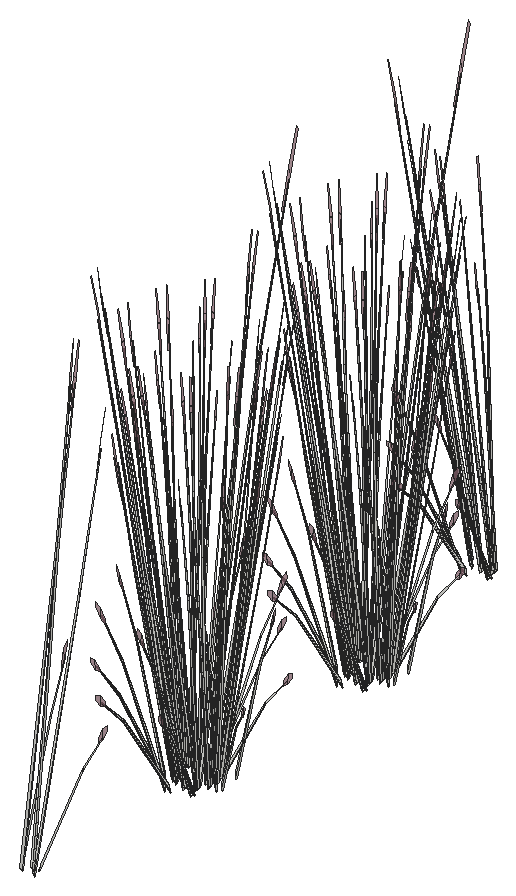
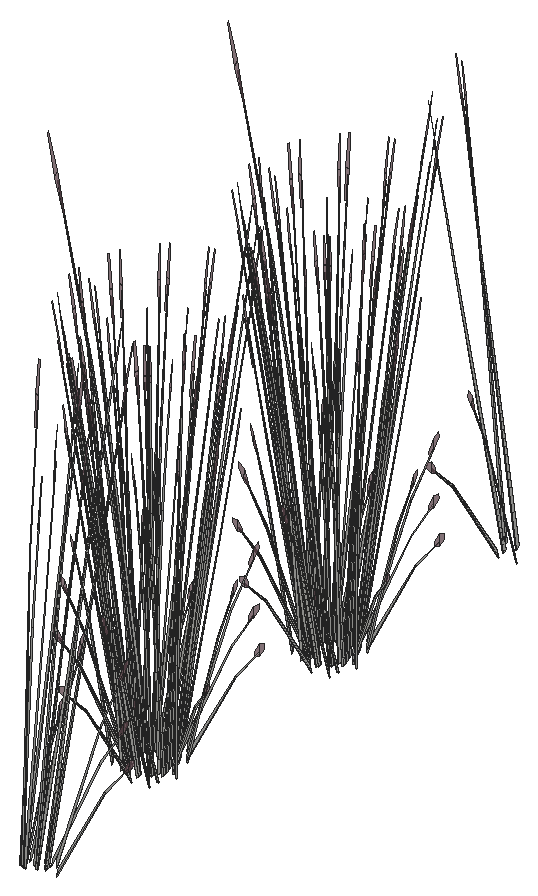
# SketchUp Ruby script. Lengths in inches.
U = 1.inch
M = Sketchup.active_model
def pt(a) = Geom::Point3d.new(a.map { |v| v * U })
def face(e, loops, mat)
  f = e.add_face(loops[0].map { |a| pt(a) })
  loops[1..].each { |l| e.add_face(l.map { |a| pt(a) }).erase! }
  f.material = f.back_material = mat if mat
  f
end
# faces: each face lists its corners as indices into pts; further lists are holes
def faces(e, pts, list, mat = nil) = list.each { |f| face(e, (f[0].is_a?(Array) ? f : [f]).map { |l| l.map { |i| pts[i] } }, mat) }
# xy, xz, yz: faces in a plane at the given z, y or x. An outline is a flat list of corners, or four numbers for a rectangle; further outlines are holes
def ring(l) = l.size == 4 ? [[l[0], l[1]], [l[2], l[1]], [l[2], l[3]], [l[0], l[3]]] : l.each_slice(2).to_a
def flat(e, list, mat, &to3) = list.each { |f| face(e, (f[0].is_a?(Array) ? f : [f]).map { |l| ring(l).map { |u, v| to3.(u, v) } }, mat) }
def xy(e, z, list, mat = nil) = flat(e, list, mat) { |x, y| [x, y, z] }
def xz(e, y, list, mat = nil) = flat(e, list, mat) { |x, z| [x, y, z] }
def yz(e, x, list, mat = nil) = flat(e, list, mat) { |y, z| [x, y, z] }
def lines(e, pts, list) = list.each { |a, b| e.add_line(pt(pts[a]), pt(pts[b])) }
# prism: a flat outline (further loops are holes) pulled along v
def prism(e, loops, v, mat = nil)
  f = face(e, loops, mat); d = Geom::Vector3d.new(v.map { |x| x * U })
  f.pushpull(f.normal.samedirection?(d) ? d.length : -d.length)
end
def box(e, o, s, mat = nil) = prism(e, [[o, [o[0] + s[0], o[1], o[2]], [o[0] + s[0], o[1] + s[1], o[2]], [o[0], o[1] + s[1], o[2]]]], [0, 0, s[2]], mat)
def at(x, y, z, deg = 0) = Geom::Transformation.translation(pt([x, y, z])) * Geom::Transformation.rotation(ORIGIN, Z_AXIS, deg.degrees)
def axes(o, x, y, z) = Geom::Transformation.new([*x, 0, *y, 0, *z, 0, *pt(o).to_a, 1])
def part(name) = M.definitions.add(name)
# library, detail: a bought-in or finely detailed component or shape, given as its bounding box
def library(name, o, s) = part(name).tap { |d| box(d.entities, o, s) }
def detail(e, o, s) = box(e.add_group.entities, o, s)
def put(e, d, t, mat = nil) = e.add_instance(d, t).tap { |i| i.material = mat if mat }
def group(e, t, mat = nil) = e.add_group.tap { |g| g.transformation = t; g.material = mat if mat }.entities
root = M.entities
M.materials.add("LightPink_Translucent").color = [144, 107, 117]
M.materials["LightPink_Translucent"].alpha = 0.75
c1 = part("blade")
p = [[2.15,0.21,22],[0,0.17,0],[0.09,0.45,0],[2.18,0.31,22],[2.29,0.31,22],[0.38,0.45,0],
  [2.48,0.24,33],[2.49,0.24,33],[2.48,0.22,33]]
faces(c1.entities,p,[[0,1,2,3],[4,5,2,3],[6,3,4,7],[8,0,3,6]])
c2 = part("seeds")
p = [[0.3,-0.1,1.38],[-0.01,-0.03,1.59],[-0.01,-0.03,0.03],[0.14,-0.07,-0.07],[0.29,-0.03,3],[0.15,0.01,3.11]]
faces(c2.entities,p,[[0,1,2,3],[1,0,4,5]],"LightPink_Translucent")
c3 = part("blade with seeds")
put(c3.entities,c1,at(0,0,0))
put(c3.entities,c2,axes([2.4,0.25,30.99],[1.5799,-0.05474,1.17369],[-0.12525,1.92788,0.29478],[-0.07173,-0.02425,1.56792]))
put(root,c3,axes([400.95,122.74,5.4],[0.3879,0.02311,-0.13498],[-0.0106,0.43749,-0.74919],[-0.02694,0.1685,1.13838]))
put(root,c3,axes([401.67,123.23,5.03],[0.34538,-0.21713,-0.1216],[0.16972,0.38536,-0.67495],[0.04557,0.16239,1.02557]))
put(root,c3,axes([401.77,123.37,5.0625],[-0.34777,-0.12192,0.53283],[0.11892,-0.40083,0.43934],[0.0209,0.15763,1.10256]))
put(root,c3,axes([400.125,123.9,4.71],[0.04004,-0.02816,1.77383],[0.33095,0.18728,-0.16761],[-0.00778,0.15594,0.31391]))
put(root,c3,axes([401.58,124.09,4.72],[0.04474,0.0751,1.74944],[0.36104,0.0295,-0.27667],[0.03631,0.16562,0.14031]))
put(root,c3,axes([401.89,138.91,4.72],[-0.05398,-0.06539,1.74944],[-0.36026,0.04145,-0.27667],[-0.0575,-0.15639,0.14031]))
put(root,c3,axes([403.51,139.71,4.72],[-0.00341,-0.09282,1.74944],[-0.28775,-0.26825,-0.27667],[0.04449,-0.16261,0.14031]))
put(root,c3,axes([403.43,139.375,4.71],[-0.03584,0.03562,1.77383],[-0.35118,-0.12018,-0.16761],[-0.01271,-0.15545,0.31391]))
put(root,c3,axes([401.52,138.69,4.71],[-0.00658,0.0559,1.77383],[-0.32474,0.20287,-0.16761],[-0.09556,-0.1037,0.31391]))
put(root,c3,axes([401.45,139.68,5.09],[0.39316,-0.11987,0.53763],[0.06823,0.47021,0.4433],[-0.09247,-0.13858,1.11249]))
put(root,c3,axes([402.34,139.77,4.73],[0.34777,0.12192,0.48003],[-0.11892,0.40083,0.3958],[-0.0209,-0.15763,0.9933]))
put(root,c3,axes([402.4375,139.92,5.03],[-0.34538,0.21713,-0.1216],[-0.16972,-0.38536,-0.67495],[-0.04557,-0.16239,1.02557]))
put(root,c3,axes([403.15,140.4,5.03],[-0.3879,-0.02311,-0.1216],[0.0106,-0.43749,-0.67495],[0.02694,-0.1685,1.02557]))
put(root,c3,axes([402.43,139.74,4.73],[0.26007,-0.1585,0.0643],[0.12729,0.28902,0.50621],[-0.02512,-0.1274,0.77189]))
put(root,c3,axes([401.54,139.79,4.73],[0.16041,-0.29625,0.0643],[0.22843,0.17248,0.50621],[-0.07385,-0.09498,0.77189]))
put(root,c3,axes([402.33,140.07,5.05],[-0.1064,0.35863,0.35414],[-0.31043,-0.1046,-0.4572],[-0.02846,-0.14439,0.87481]))
put(root,c3,axes([403.125,140.22,4.73],[0.25132,0.3182,0.48003],[-0.2669,0.27442,0.3958],[0.04636,-0.14929,0.9933]))
put(root,c3,axes([401.61,139.76,5.43],[-0.23555,0.44708,-0.13619],[-0.34112,-0.25757,-0.75594],[-0.11858,-0.12631,1.14864]))
put(root,c3,axes([403.22,140.25,4.73],[0.29004,0.02173,0.0643],[-0.00795,0.32812,0.50621],[0.03035,-0.12569,0.77189]))
put(root,c3,axes([403,140.47,5.05],[-0.23881,0.24554,0.35414],[-0.22606,-0.28036,-0.4572],[0.0344,-0.14245,0.87481]))
put(root,c3,axes([400.71,139.625,4.72],[-0.07594,-0.00329,1.74944],[-0.24177,0.32918,-0.27667],[-0.129,-0.06726,0.14031]))
put(root,c3,axes([403.58,141.26,5.03],[-0.32648,-0.25715,-0.1216],[0.18809,-0.3724,-0.67495],[0.09224,-0.12945,1.02557]))
put(root,c3,axes([401.59,140.125,5.05],[0.05451,0.37564,0.35414],[-0.31161,0.09919,-0.4572],[-0.0837,-0.10765,0.87481]))
put(root,c3,axes([400.65,140.37,5.09],[0.29147,-0.34417,0.53763],[0.25138,0.3655,0.4433],[-0.13675,-0.06349,1.11249]))
put(root,c3,axes([404.38,141.15,4.71],[-0.0461,-0.00354,1.77383],[-0.19143,-0.37951,-0.16761],[0.07688,-0.12478,0.31391]))
put(root,c3,axes([400.78,140.37,4.73],[0.01777,-0.35463,0.0643],[0.26836,0.00972,0.50621],[-0.1028,-0.03711,0.77189]))
put(root,c3,axes([403.42,141.23,5.05],[-0.30722,0.06665,0.35414],[-0.08112,-0.381,-0.4572],[0.08804,-0.10234,0.87481]))
put(root,c3,axes([403.7,141.17,4.73],[0.2423,0.19613,0.0643],[-0.14107,0.2793,0.50621],[0.07768,-0.0903,0.77189]))
put(root,c3,axes([403.63,141.09,4.73],[0.08753,0.42921,0.48003],[-0.34336,0.07449,0.3958],[0.1012,-0.10094,0.9933]))
put(root,c3,axes([404.55,141.61,4.72],[0.04898,-0.07104,1.74944],[-0.06269,-0.43574,-0.27667],[0.12289,-0.08262,0.14031]))
put(root,c3,axes([400.42,139.91,4.71],[0.02617,0.04654,1.77383],[-0.12614,0.41836,-0.16761],[-0.12775,0.00303,0.31391]))
put(root,c3,axes([400.97,140.63,5.05],[0.20082,0.29199,0.35414],[-0.2293,0.2764,-0.4572],[-0.1165,-0.04206,0.87481]))
put(root,c3,axes([400.91,140.45,5.03],[-0.0189,0.47427,-0.1216],[-0.35781,-0.01296,-0.67495],[-0.13781,-0.03295,1.02557]))
put(root,c3,axes([403.59,142.27,5.03],[-0.17758,-0.42229,-0.1216],[0.31518,-0.20752,-0.67495],[0.13282,-0.05572,1.02557]))
put(root,c3,axes([403.47,142.14,5.05],[-0.29332,-0.1301,0.35414],[0.08555,-0.37955,-0.4572],[0.11809,-0.0348,0.87481]))
put(root,c3,axes([400.4,141.45,4.73],[0.09971,-0.42522,0.48003],[0.32782,0.1454,0.3958],[-0.12892,0.02555,0.9933]))
put(root,c3,axes([400.37,141.33,4.73],[-0.12963,-0.31798,0.0643],[0.23638,-0.15564,0.50621],[-0.1042,0.03071,0.77189]))
put(root,c3,axes([403.73,142.26,4.73],[0.12963,0.31798,0.0643],[-0.23638,0.15564,0.50621],[0.1042,-0.03071,0.77189]))
put(root,c3,axes([403.71,142.15,4.73],[-0.09971,0.42522,0.48003],[-0.32782,-0.1454,0.3958],[0.12892,-0.02555,0.9933]))
put(root,c3,axes([400.64,141.45,5.05],[0.29332,0.1301,0.35414],[-0.08555,0.37955,-0.4572],[-0.11809,0.0348,0.87481]))
put(root,c3,axes([404.3,143.52,4.71],[-0.03191,-0.04083,1.77383],[0.06981,-0.43764,-0.16761],[0.12571,-0.02796,0.31391]))
put(root,c3,axes([400.14,141.75,4.72],[-0.05763,0.06055,1.74944],[0.0049,0.44239,-0.27667],[-0.13211,0.05753,0.14031]))
put(root,c3,axes([400.51,141.33,5.03],[0.17758,0.42229,-0.1216],[-0.31518,0.20752,-0.67495],[-0.13282,0.05572,1.02557]))
put(root,c3,axes([403.19,143.15,5.03],[0.0189,-0.47427,-0.1216],[0.35781,0.01296,-0.67495],[0.13781,0.03295,1.02557]))
put(root,c3,axes([403.14,142.96,5.05],[-0.20082,-0.29199,0.35414],[0.2293,-0.2764,-0.4572],[0.1165,0.04206,0.87481]))
put(root,c3,axes([403.5,142.86,4.72],[0.07571,-0.00789,1.74944],[0.20767,-0.36231,-0.27667],[0.13467,0.04783,0.14031]))
put(root,c3,axes([400.47,142.51,4.73],[-0.08753,-0.42921,0.48003],[0.34336,-0.07449,0.3958],[-0.1012,0.10094,0.9933]))
put(root,c3,axes([400.41,142.42,4.73],[-0.2423,-0.19613,0.0643],[0.14107,-0.2793,0.50621],[-0.07768,0.0903,0.77189]))
put(root,c3,axes([400.6875,142.36,5.05],[0.30722,-0.06665,0.35414],[0.08112,0.381,-0.4572],[-0.08804,0.10234,0.87481]))
put(root,c3,axes([399.5,142.19,4.71],[0.04504,0.01251,1.77383],[0.13934,0.41205,-0.16761],[-0.0922,0.10815,0.31391]))
put(root,c3,axes([403.32,143.22,4.73],[-0.01777,0.35463,0.0643],[-0.26836,-0.00972,0.50621],[0.1028,0.03711,0.77189]))
put(root,c3,axes([403.34,143.11,4.73],[-0.26024,0.30729,0.48003],[-0.22444,-0.32634,0.3958],[0.1221,0.05668,0.9933]))
put(root,c3,axes([399.99,143.45,5.65],[0.31145,0.12449,-0.06488],[-0.0958,0.38314,-0.29416],[-0.05094,0.05817,0.97024]))
put(root,c3,axes([402.52,143.47,5.05],[-0.05451,-0.37564,0.35414],[0.31161,-0.09919,-0.4572],[0.0837,0.10765,0.87481]))
put(root,c3,axes([402.72,141.31,4.47],[-0.30498,-0.24231,1.38283],[0.32203,-0.37727,0.59665],[0.0984,0.22736,1.33663]))
put(root,c3,axes([400.53,142.33,5.03],[0.32648,0.25715,-0.1216],[-0.18809,0.3724,-0.67495],[-0.09224,0.12945,1.02557]))
put(root,c3,axes([402.49,143.66,5.03],[0.21031,-0.39918,-0.1216],[0.30457,0.22997,-0.67495],[0.10587,0.11278,1.02557]))
put(root,c3,axes([401.1,143.12,5.05],[0.23881,-0.24554,0.35414],[0.22606,0.28036,-0.4572],[-0.0344,0.14245,0.87481]))
put(root,c3,axes([402.21,143.99,4.71],[0.00104,-0.05646,1.77383],[0.30246,-0.2491,-0.16761],[0.10506,0.08891,0.31391]))
put(root,c3,axes([400.88,143.35,4.73],[-0.29004,-0.02173,0.0643],[0.00795,-0.32812,0.50621],[-0.03035,0.12569,0.77189]))
put(root,c3,axes([400.98,143.375,4.73],[-0.25132,-0.3182,0.48003],[0.2669,-0.27442,0.3958],[-0.04636,0.14929,0.9933]))
put(root,c3,axes([401.77,143.53,5.05],[0.1064,-0.35863,0.35414],[0.31043,0.1046,-0.4572],[0.02846,0.14439,0.87481]))
put(root,c3,axes([402.56,143.81,4.73],[-0.16041,0.29625,0.0643],[-0.22843,-0.17248,0.50621],[0.07385,0.09498,0.77189]))
put(root,c3,axes([402.1875,144.81,5.65],[0.2439,-0.26754,-0.06488],[0.22348,0.29302,-0.29416],[0.01573,0.08303,0.97024]))
put(root,c3,axes([402.63,143.72,4.73],[-0.35104,0.10702,0.48003],[-0.06092,-0.41983,0.3958],[0.08256,0.12373,0.9933]))
put(root,c3,axes([401.67,143.85,4.73],[-0.26007,0.1585,0.0643],[-0.12729,-0.28902,0.50621],[0.02512,0.1274,0.77189]))
put(root,c3,axes([400.15,143.4,4.72],[-0.00877,0.09229,1.74944],[0.24897,0.32105,-0.27667],[-0.06518,0.15182,0.14031]))
put(root,c3,axes([400.95,143.19,5.4],[0.3879,0.02311,-0.13498],[-0.0106,0.43749,-0.74919],[-0.02694,0.1685,1.13838]))
put(root,c3,axes([401.67,143.68,5.03],[0.34538,-0.21713,-0.1216],[0.16972,0.38536,-0.67495],[0.04557,0.16239,1.02557]))
put(root,c3,axes([401.77,143.82,5.0625],[-0.34777,-0.12192,0.53283],[0.11892,-0.40083,0.43934],[0.0209,0.15763,1.10256]))
put(root,c3,axes([400.125,144.34,4.71],[0.04004,-0.02816,1.77383],[0.33095,0.18728,-0.16761],[-0.00778,0.15594,0.31391]))
put(root,c3,axes([401.58,144.54,4.72],[0.04474,0.0751,1.74944],[0.36104,0.0295,-0.27667],[0.03631,0.16562,0.14031]))
put(root,c3,axes([401.89,158.6,4.72],[-0.05398,-0.06539,1.74944],[-0.36026,0.04145,-0.27667],[-0.0575,-0.15639,0.14031]))
put(root,c3,axes([403.51,159.4,4.72],[-0.00341,-0.09282,1.74944],[-0.28775,-0.26825,-0.27667],[0.04449,-0.16261,0.14031]))
put(root,c3,axes([403.43,159.07,4.71],[-0.03584,0.03562,1.77383],[-0.35118,-0.12018,-0.16761],[-0.01271,-0.15545,0.31391]))
put(root,c3,axes([401.52,158.39,4.71],[-0.00658,0.0559,1.77383],[-0.32474,0.20287,-0.16761],[-0.09556,-0.1037,0.31391]))
put(root,c3,axes([401.45,159.38,5.09],[0.39316,-0.11987,0.53763],[0.06823,0.47021,0.4433],[-0.09247,-0.13858,1.11249]))
put(root,c3,axes([402.34,159.47,4.73],[0.34777,0.12192,0.48003],[-0.11892,0.40083,0.3958],[-0.0209,-0.15763,0.9933]))
put(root,c3,axes([402.4375,159.61,5.03],[-0.34538,0.21713,-0.1216],[-0.16972,-0.38536,-0.67495],[-0.04557,-0.16239,1.02557]))
put(root,c3,axes([403.15,160.1,5.03],[-0.3879,-0.02311,-0.1216],[0.0106,-0.43749,-0.67495],[0.02694,-0.1685,1.02557]))
put(root,c3,axes([402.43,159.4375,4.73],[0.26007,-0.1585,0.0643],[0.12729,0.28902,0.50621],[-0.02512,-0.1274,0.77189]))
put(root,c3,axes([401.54,159.48,4.73],[0.16041,-0.29625,0.0643],[0.22843,0.17248,0.50621],[-0.07385,-0.09498,0.77189]))
put(root,c3,axes([402.33,159.76,5.05],[-0.1064,0.35863,0.35414],[-0.31043,-0.1046,-0.4572],[-0.02846,-0.14439,0.87481]))
put(root,c3,axes([403.125,159.91,4.73],[0.25132,0.3182,0.48003],[-0.2669,0.27442,0.3958],[0.04636,-0.14929,0.9933]))
put(root,c3,axes([401.61,159.45,5.43],[-0.23555,0.44708,-0.13619],[-0.34112,-0.25757,-0.75594],[-0.11858,-0.12631,1.14864]))
put(root,c3,axes([403.22,159.94,4.73],[0.29004,0.02173,0.0643],[-0.00795,0.32812,0.50621],[0.03035,-0.12569,0.77189]))
put(root,c3,axes([403,160.17,5.05],[-0.23881,0.24554,0.35414],[-0.22606,-0.28036,-0.4572],[0.0344,-0.14245,0.87481]))
put(root,c3,axes([400.71,159.32,4.72],[-0.07594,-0.00329,1.74944],[-0.24177,0.32918,-0.27667],[-0.129,-0.06726,0.14031]))
put(root,c3,axes([403.58,160.96,5.03],[-0.32648,-0.25715,-0.1216],[0.18809,-0.3724,-0.67495],[0.09224,-0.12945,1.02557]))
put(root,c3,axes([401.59,159.82,5.05],[0.05451,0.37564,0.35414],[-0.31161,0.09919,-0.4572],[-0.0837,-0.10765,0.87481]))
put(root,c3,axes([400.65,160.07,5.09],[0.29147,-0.34417,0.53763],[0.25138,0.3655,0.4433],[-0.13675,-0.06349,1.11249]))
put(root,c3,axes([404.38,160.85,4.71],[-0.0461,-0.00354,1.77383],[-0.19143,-0.37951,-0.16761],[0.07688,-0.12478,0.31391]))
put(root,c3,axes([400.78,160.0625,4.73],[0.01777,-0.35463,0.0643],[0.26836,0.00972,0.50621],[-0.1028,-0.03711,0.77189]))
put(root,c3,axes([403.42,160.92,5.05],[-0.30722,0.06665,0.35414],[-0.08112,-0.381,-0.4572],[0.08804,-0.10234,0.87481]))
put(root,c3,axes([403.7,160.86,4.73],[0.2423,0.19613,0.0643],[-0.14107,0.2793,0.50621],[0.07768,-0.0903,0.77189]))
put(root,c3,axes([403.63,160.78,4.73],[0.08753,0.42921,0.48003],[-0.34336,0.07449,0.3958],[0.1012,-0.10094,0.9933]))
put(root,c3,axes([404.55,161.3,4.72],[0.04898,-0.07104,1.74944],[-0.06269,-0.43574,-0.27667],[0.12289,-0.08262,0.14031]))
put(root,c3,axes([400.42,159.6,4.71],[0.02617,0.04654,1.77383],[-0.12614,0.41836,-0.16761],[-0.12775,0.00303,0.31391]))
put(root,c3,axes([400.97,160.33,5.05],[0.20082,0.29199,0.35414],[-0.2293,0.2764,-0.4572],[-0.1165,-0.04206,0.87481]))
put(root,c3,axes([400.91,160.14,5.03],[-0.0189,0.47427,-0.1216],[-0.35781,-0.01296,-0.67495],[-0.13781,-0.03295,1.02557]))
put(root,c3,axes([403.59,161.96,5.03],[-0.17758,-0.42229,-0.1216],[0.31518,-0.20752,-0.67495],[0.13282,-0.05572,1.02557]))
put(root,c3,axes([403.47,161.84,5.05],[-0.29332,-0.1301,0.35414],[0.08555,-0.37955,-0.4572],[0.11809,-0.0348,0.87481]))
put(root,c3,axes([400.4,161.14,4.73],[0.09971,-0.42522,0.48003],[0.32782,0.1454,0.3958],[-0.12892,0.02555,0.9933]))
put(root,c3,axes([400.37,161.03,4.73],[-0.12963,-0.31798,0.0643],[0.23638,-0.15564,0.50621],[-0.1042,0.03071,0.77189]))
put(root,c3,axes([403.73,161.95,4.73],[0.12963,0.31798,0.0643],[-0.23638,0.15564,0.50621],[0.1042,-0.03071,0.77189]))
put(root,c3,axes([403.71,161.84,4.73],[-0.09971,0.42522,0.48003],[-0.32782,-0.1454,0.3958],[0.12892,-0.02555,0.9933]))
put(root,c3,axes([400.64,161.15,5.05],[0.29332,0.1301,0.35414],[-0.08555,0.37955,-0.4572],[-0.11809,0.0348,0.87481]))
put(root,c3,axes([404.3,163.22,4.71],[-0.03191,-0.04083,1.77383],[0.06981,-0.43764,-0.16761],[0.12571,-0.02796,0.31391]))
put(root,c3,axes([400.14,161.44,4.72],[-0.05763,0.06055,1.74944],[0.0049,0.44239,-0.27667],[-0.13211,0.05753,0.14031]))
put(root,c3,axes([400.51,161.02,5.03],[0.17758,0.42229,-0.1216],[-0.31518,0.20752,-0.67495],[-0.13282,0.05572,1.02557]))
put(root,c3,axes([403.19,162.84,5.03],[0.0189,-0.47427,-0.1216],[0.35781,0.01296,-0.67495],[0.13781,0.03295,1.02557]))
put(root,c3,axes([403.14,162.65,5.05],[-0.20082,-0.29199,0.35414],[0.2293,-0.2764,-0.4572],[0.1165,0.04206,0.87481]))
put(root,c3,axes([403.5,162.56,4.72],[0.07571,-0.00789,1.74944],[0.20767,-0.36231,-0.27667],[0.13467,0.04783,0.14031]))
put(root,c3,axes([400.47,162.2,4.73],[-0.08753,-0.42921,0.48003],[0.34336,-0.07449,0.3958],[-0.1012,0.10094,0.9933]))
put(root,c3,axes([400.41,162.12,4.73],[-0.2423,-0.19613,0.0643],[0.14107,-0.2793,0.50621],[-0.07768,0.0903,0.77189]))
put(root,c3,axes([400.6875,162.06,5.05],[0.30722,-0.06665,0.35414],[0.08112,0.381,-0.4572],[-0.08804,0.10234,0.87481]))
put(root,c3,axes([399.5,161.89,4.71],[0.04504,0.01251,1.77383],[0.13934,0.41205,-0.16761],[-0.0922,0.10815,0.31391]))
put(root,c3,axes([403.32,162.92,4.73],[-0.01777,0.35463,0.0643],[-0.26836,-0.00972,0.50621],[0.1028,0.03711,0.77189]))
put(root,c3,axes([403.34,162.81,4.73],[-0.26024,0.30729,0.48003],[-0.22444,-0.32634,0.3958],[0.1221,0.05668,0.9933]))
put(root,c3,axes([399.99,163.14,5.65],[0.31145,0.12449,-0.06488],[-0.0958,0.38314,-0.29416],[-0.05094,0.05817,0.97024]))
put(root,c3,axes([402.52,163.16,5.05],[-0.05451,-0.37564,0.35414],[0.31161,-0.09919,-0.4572],[0.0837,0.10765,0.87481]))
put(root,c3,axes([402.72,161,4.47],[-0.30498,-0.24231,1.38283],[0.32203,-0.37727,0.59665],[0.0984,0.22736,1.33663]))
put(root,c3,axes([400.53,162.02,5.03],[0.32648,0.25715,-0.1216],[-0.18809,0.3724,-0.67495],[-0.09224,0.12945,1.02557]))
put(root,c3,axes([402.49,163.36,5.03],[0.21031,-0.39918,-0.1216],[0.30457,0.22997,-0.67495],[0.10587,0.11278,1.02557]))
put(root,c3,axes([401.1,162.82,5.05],[0.23881,-0.24554,0.35414],[0.22606,0.28036,-0.4572],[-0.0344,0.14245,0.87481]))
put(root,c3,axes([402.21,163.6875,4.71],[0.00104,-0.05646,1.77383],[0.30246,-0.2491,-0.16761],[0.10506,0.08891,0.31391]))
put(root,c3,axes([400.88,163.04,4.73],[-0.29004,-0.02173,0.0643],[0.00795,-0.32812,0.50621],[-0.03035,0.12569,0.77189]))
put(root,c3,axes([400.98,163.07,4.73],[-0.25132,-0.3182,0.48003],[0.2669,-0.27442,0.3958],[-0.04636,0.14929,0.9933]))
put(root,c3,axes([401.77,163.22,5.05],[0.1064,-0.35863,0.35414],[0.31043,0.1046,-0.4572],[0.02846,0.14439,0.87481]))
put(root,c3,axes([402.56,163.5,4.73],[-0.16041,0.29625,0.0643],[-0.22843,-0.17248,0.50621],[0.07385,0.09498,0.77189]))
put(root,c3,axes([402.1875,164.5,5.65],[0.2439,-0.26754,-0.06488],[0.22348,0.29302,-0.29416],[0.01573,0.08303,0.97024]))
put(root,c3,axes([402.63,163.42,4.73],[-0.35104,0.10702,0.48003],[-0.06092,-0.41983,0.3958],[0.08256,0.12373,0.9933]))
put(root,c3,axes([401.67,163.55,4.73],[-0.26007,0.1585,0.0643],[-0.12729,-0.28902,0.50621],[0.02512,0.1274,0.77189]))
put(root,c3,axes([400.15,163.09,4.72],[-0.00877,0.09229,1.74944],[0.24897,0.32105,-0.27667],[-0.06518,0.15182,0.14031]))
put(root,c3,axes([400.95,162.88,5.4],[0.3879,0.02311,-0.13498],[-0.0106,0.43749,-0.74919],[-0.02694,0.1685,1.13838]))
put(root,c3,axes([401.67,163.37,5.03],[0.34538,-0.21713,-0.1216],[0.16972,0.38536,-0.67495],[0.04557,0.16239,1.02557]))
put(root,c3,axes([401.77,163.52,5.0625],[-0.34777,-0.12192,0.53283],[0.11892,-0.40083,0.43934],[0.0209,0.15763,1.10256]))
put(root,c3,axes([400.125,164.04,4.71],[0.04004,-0.02816,1.77383],[0.33095,0.18728,-0.16761],[-0.00778,0.15594,0.31391]))
put(root,c3,axes([401.58,164.23,4.72],[0.04474,0.0751,1.74944],[0.36104,0.0295,-0.27667],[0.03631,0.16562,0.14031]))
put(root,c3,axes([398.69,176.86,4.72],[-0.05398,-0.06539,1.74944],[-0.36026,0.04145,-0.27667],[-0.0575,-0.15639,0.14031]))
put(root,c3,axes([400.3125,177.66,4.72],[-0.00341,-0.09282,1.74944],[-0.28775,-0.26825,-0.27667],[0.04449,-0.16261,0.14031]))
put(root,c3,axes([400.23,177.33,4.71],[-0.03584,0.03562,1.77383],[-0.35118,-0.12018,-0.16761],[-0.01271,-0.15545,0.31391]))
put(root,c3,axes([398.32,176.65,4.71],[-0.00658,0.0559,1.77383],[-0.32474,0.20287,-0.16761],[-0.09556,-0.1037,0.31391]))
put(root,c3,axes([398.25,177.64,5.09],[0.39316,-0.11987,0.53763],[0.06823,0.47021,0.4433],[-0.09247,-0.13858,1.11249]))
put(root,c3,axes([399.14,177.73,4.73],[0.34777,0.12192,0.48003],[-0.11892,0.40083,0.3958],[-0.0209,-0.15763,0.9933]))
put(root,c3,axes([399.24,177.87,5.03],[-0.34538,0.21713,-0.1216],[-0.16972,-0.38536,-0.67495],[-0.04557,-0.16239,1.02557]))
put(root,c3,axes([399.96,178.36,5.03],[-0.3879,-0.02311,-0.1216],[0.0106,-0.43749,-0.67495],[0.02694,-0.1685,1.02557]))
put(root,c3,axes([399.23,177.69,4.73],[0.26007,-0.1585,0.0643],[0.12729,0.28902,0.50621],[-0.02512,-0.1274,0.77189]))
put(root,c3,axes([398.34,177.74,4.73],[0.16041,-0.29625,0.0643],[0.22843,0.17248,0.50621],[-0.07385,-0.09498,0.77189]))
put(root,c3,axes([399.14,178.02,5.05],[-0.1064,0.35863,0.35414],[-0.31043,-0.1046,-0.4572],[-0.02846,-0.14439,0.87481]))
put(root,c3,axes([399.93,178.17,4.73],[0.25132,0.3182,0.48003],[-0.2669,0.27442,0.3958],[0.04636,-0.14929,0.9933]))
put(root,c3,axes([398.41,177.71,5.43],[-0.23555,0.44708,-0.13619],[-0.34112,-0.25757,-0.75594],[-0.11858,-0.12631,1.14864]))
put(root,c3,axes([400.02,178.2,4.73],[0.29004,0.02173,0.0643],[-0.00795,0.32812,0.50621],[0.03035,-0.12569,0.77189]))
put(root,c3,axes([399.81,178.42,5.05],[-0.23881,0.24554,0.35414],[-0.22606,-0.28036,-0.4572],[0.0344,-0.14245,0.87481]))
put(root,c3,axes([397.51,177.58,4.72],[-0.07594,-0.00329,1.74944],[-0.24177,0.32918,-0.27667],[-0.129,-0.06726,0.14031]))
